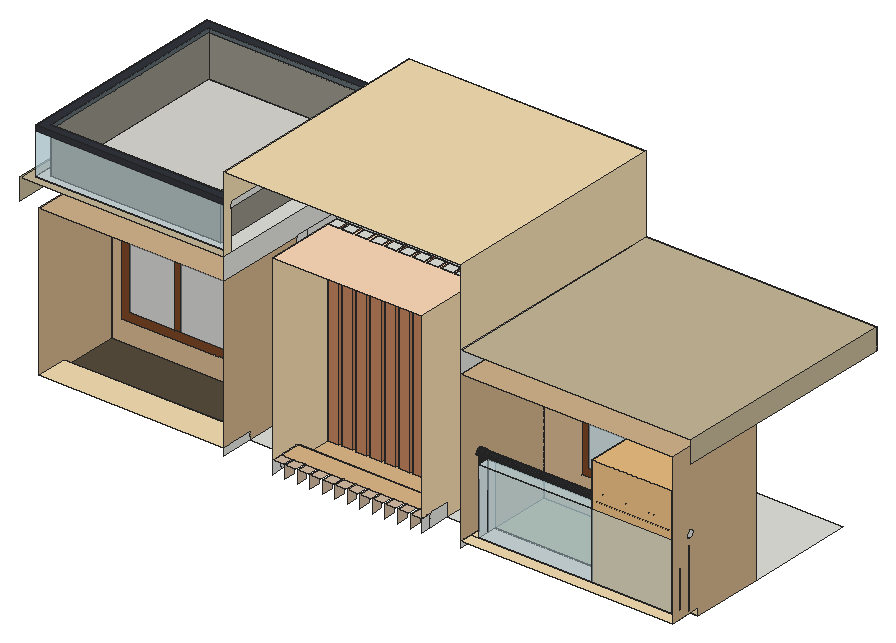
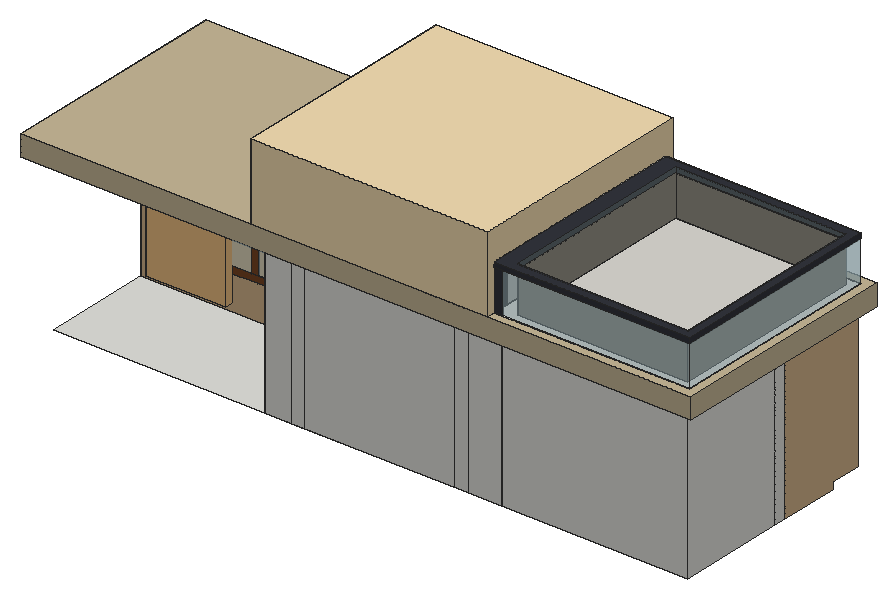
# SketchUp Ruby script. Lengths in inches.
U = 1.inch
M = Sketchup.active_model
def pt(a) = Geom::Point3d.new(a.map { |v| v * U })
def face(e, loops, mat)
  f = e.add_face(loops[0].map { |a| pt(a) })
  loops[1..].each { |l| e.add_face(l.map { |a| pt(a) }).erase! }
  f.material = f.back_material = mat if mat
  f
end
# faces: each face lists its corners as indices into pts; further lists are holes
def faces(e, pts, list, mat = nil) = list.each { |f| face(e, (f[0].is_a?(Array) ? f : [f]).map { |l| l.map { |i| pts[i] } }, mat) }
# xy, xz, yz: faces in a plane at the given z, y or x. An outline is a flat list of corners, or four numbers for a rectangle; further outlines are holes
def ring(l) = l.size == 4 ? [[l[0], l[1]], [l[2], l[1]], [l[2], l[3]], [l[0], l[3]]] : l.each_slice(2).to_a
def flat(e, list, mat, &to3) = list.each { |f| face(e, (f[0].is_a?(Array) ? f : [f]).map { |l| ring(l).map { |u, v| to3.(u, v) } }, mat) }
def xy(e, z, list, mat = nil) = flat(e, list, mat) { |x, y| [x, y, z] }
def xz(e, y, list, mat = nil) = flat(e, list, mat) { |x, z| [x, y, z] }
def yz(e, x, list, mat = nil) = flat(e, list, mat) { |y, z| [x, y, z] }
def lines(e, pts, list) = list.each { |a, b| e.add_line(pt(pts[a]), pt(pts[b])) }
# prism: a flat outline (further loops are holes) pulled along v
def prism(e, loops, v, mat = nil)
  f = face(e, loops, mat); d = Geom::Vector3d.new(v.map { |x| x * U })
  f.pushpull(f.normal.samedirection?(d) ? d.length : -d.length)
end
def box(e, o, s, mat = nil) = prism(e, [[o, [o[0] + s[0], o[1], o[2]], [o[0] + s[0], o[1] + s[1], o[2]], [o[0], o[1] + s[1], o[2]]]], [0, 0, s[2]], mat)
def at(x, y, z, deg = 0) = Geom::Transformation.translation(pt([x, y, z])) * Geom::Transformation.rotation(ORIGIN, Z_AXIS, deg.degrees)
def axes(o, x, y, z) = Geom::Transformation.new([*x, 0, *y, 0, *z, 0, *pt(o).to_a, 1])
def part(name) = M.definitions.add(name)
# library, detail: a bought-in or finely detailed component or shape, given as its bounding box
def library(name, o, s) = part(name).tap { |d| box(d.entities, o, s) }
def detail(e, o, s) = box(e.add_group.entities, o, s)
def put(e, d, t, mat = nil) = e.add_instance(d, t).tap { |i| i.material = mat if mat }
def group(e, t, mat = nil) = e.add_group.tap { |g| g.transformation = t; g.material = mat if mat }.entities
root = M.entities
M.materials.add("[0027_PeachPuff]").color = [255, 218, 185]
M.materials.add("[0034_Wheat]").color = [245, 222, 179]
M.materials.add("[0035_Tan]").color = [210, 180, 140]
M.materials.add("[0036_BurlyWood]1").color = [222, 184, 135]
M.materials.add("[Carpet Diamond Olive]").color = [87, 77, 61]
M.materials.add("[Formica Beige]").color = [247, 219, 174]
M.materials.add("[Formica Graystone]").color = [149, 146, 135]
M.materials.add("[Formica Laminate Dark]").color = [50, 53, 60]
M.materials.add("[Formica Laminate Light]").color = [213, 189, 164]
M.materials.add("[Formica Speckled Grey]").color = [94, 105, 111]
M.materials.add("[Quartz Light Brown]").color = [199, 184, 152]
M.materials.add("[Terrazzo Tile Light]").color = [219, 217, 210]
M.materials.add("[Tile Ceramic Natural]").color = [189, 180, 134]
M.materials.add("[Translucent Glass Gray]").color = [191, 191, 191]
M.materials["[Translucent Glass Gray]"].alpha = 0.5
M.materials.add("[Translucent Glass Safety]").color = [204, 235, 244]
M.materials["[Translucent Glass Safety]"].alpha = 0.5
M.materials.add("[Wood Veneer 01]").color = [120, 70, 37]
M.materials.add("[Wood Veneer 02]").color = [190, 128, 91]
c1 = library("chau cay",[-24.34,-109.24,0],[56.46,62.58,79.69])
xy(root,4500.3125,[[646.67,397.09,752.97,971.67],[752.97,397.09,800.41,971.67],[1272.8,397.09,1313.62,971.67],[1313.62,397.09,1398.32,971.67],[800.41,515.23,836.51,548.98],
  [842.91,515.23,879.01,548.98],[888.47,515.23,924.57,548.98],[934.66,515.23,970.76,548.98],[980.66,515.23,1016.76,548.98],[1024.6,515.23,1060.7,548.98],
  [1069.41,515.23,1105.51,548.98],[1113.97,515.23,1150.07,548.98],[1159.22,515.23,1195.32,548.98],[1202.41,515.23,1228.29,548.98],[1238.51,515.23,1272.8,548.98],
  [800.41,548.98,1272.8,971.67],[58.44,584.29,646.67,623.89],[58.44,623.89,646.67,971.67],[1398.32,623.89,2069.85,971.67]])
xy(root,4500.3125,[[800.41,397.09,1272.8,397.09,1272.8,515.23,1238.51,515.23,1238.51,548.98,1228.29,548.98,1228.29,515.23,1202.41,515.23,1202.41,548.98,1195.32,548.98,1195.32,515.23,1159.22,515.23,1159.22,548.98,1150.07,548.98,1150.07,515.23,1113.97,515.23,1113.97,548.98,1105.51,548.98,1105.51,515.23,1069.41,515.23,1069.41,548.98,1060.7,548.98,1060.7,515.23,1024.6,515.23,1024.6,548.98,1016.76,548.98,1016.76,515.23,980.66,515.23,980.66,548.98,970.76,548.98,970.76,515.23,934.66,515.23,934.66,548.98,924.57,548.98,924.57,515.23,888.47,515.23,888.47,548.98,879.01,548.98,879.01,515.23,842.91,515.23,842.91,548.98,836.51,548.98,836.51,515.23,800.41,515.23]],"[0036_BurlyWood]1")
xy(root,4500.3125,[[58.44,397.09,646.67,584.29]],"[Carpet Diamond Olive]")
xy(root,4500.3125,[[1398.32,397.09,2069.85,623.89]],"[Tile Ceramic Natural]")
xy(root,4522.25,[[1424.82,334.4,2037.625,397.09],[1412.33,356.37,1409.51,356.74,1406.89,357.82,1404.64,359.55,1402.91,361.8,1401.82,364.43,1401.45,367.24,1401.82,370.06,1402.91,372.68,1404.64,374.93,1406.89,376.66,1409.51,377.75,1412.33,378.12,1415.14,377.75,1417.76,376.66,1420.02,374.93,1421.74,372.68,1422.83,370.06,1423.2,367.24,1422.83,364.43,1421.74,361.8,1420.02,359.55,1417.76,357.82,1415.14,356.74],[2049.64,356.37,2046.82,356.74,2044.2,357.82,2041.95,359.55,2040.22,361.8,2039.13,364.43,2038.76,367.24,2039.13,370.06,2040.22,372.68,2041.95,374.93,2044.2,376.66,2046.82,377.75,2049.64,378.12,2052.45,377.75,2055.08,376.66,2057.33,374.93,2059.06,372.68,2060.14,370.06,2060.51,367.24,2060.14,364.43,2059.06,361.8,2057.33,359.55,2055.08,357.82,2052.45,356.74]])
xy(root,4522.25,[[58.44,295.82,646.67,397.09],[1398.32,295.82,2069.85,334.4],[[1398.32,334.4,1424.82,397.09],[1412.33,356.37,1409.51,356.74,1406.89,357.82,1404.64,359.55,1402.91,361.8,1401.82,364.43,1401.45,367.24,1401.82,370.06,1402.91,372.68,1404.64,374.93,1406.89,376.66,1409.51,377.75,1412.33,378.12,1415.14,377.75,1417.76,376.66,1420.02,374.93,1421.74,372.68,1422.83,370.06,1423.2,367.24,1422.83,364.43,1421.74,361.8,1420.02,359.55,1417.76,357.82,1415.14,356.74]],[[2037.625,334.4,2069.85,397.09],[2049.64,356.37,2046.82,356.74,2044.2,357.82,2041.95,359.55,2040.22,361.8,2039.13,364.43,2038.76,367.24,2039.13,370.06,2040.22,372.68,2041.95,374.93,2044.2,376.66,2046.82,377.75,2049.64,378.12,2052.45,377.75,2055.08,376.66,2057.33,374.93,2059.06,372.68,2060.14,370.06,2060.51,367.24,2060.14,364.43,2059.06,361.8,2057.33,359.55,2055.08,357.82,2052.45,356.74]]],"[0034_Wheat]")
xy(root,4541.3125,[[800.41,329.94,1272.8,397.09]],"[0036_BurlyWood]1")
xy(root,4541.3125,[[800.41,295.82,834.61,329.94],[840.03,295.82,874.24,329.94],[880.03,295.82,914.24,329.94],[919.91,295.82,954.11,329.94],[959.66,295.82,993.86,329.94],
  [998.72,295.82,1032.93,329.94],[1037.47,295.82,1071.68,329.94],[1076.91,295.82,1111.11,329.94],[1117.03,295.82,1151.24,329.94],[1157.28,295.82,1191.49,329.94],
  [1197.94,295.82,1232.15,329.94],[1238.6,295.82,1272.8,329.94]],"[Formica Laminate Light]")
xy(root,4730.6875,[[1424.82,334.4,2037.625,397.09]],"[Translucent Glass Safety]")
xy(root,4752.45,[[1412.33,356.37,1415.14,356.74,1417.76,357.82,1420.02,359.55,1421.74,361.8,1422.83,364.43,1423.2,367.24,1422.83,370.06,1421.74,372.68,1421.18,373.42,1403.47,373.42,1402.91,372.68,1401.82,370.06,1401.45,367.24,1401.82,364.43,1402.91,361.8,1404.64,359.55,1406.89,357.82,1409.51,356.74],[2049.64,356.37,2052.45,356.74,2055.08,357.82,2057.33,359.55,2059.06,361.8,2060.14,364.43,2060.51,367.24,2060.14,370.06,2059.06,372.68,2058.49,373.42,2040.79,373.42,2040.22,372.68,2039.13,370.06,2038.76,367.24,2039.13,364.43,2040.22,361.8,2041.95,359.55,2044.2,357.82,2046.82,356.74],[1403.47,373.42,1421.18,373.42,1420.02,374.93,1417.76,376.66,1415.14,377.75,1412.33,378.12,1409.51,377.75,1406.89,376.66,1404.64,374.93],[2040.79,373.42,2058.49,373.42,2057.33,374.93,2055.08,376.66,2052.45,377.75,2049.64,378.12,2046.82,377.75,2044.2,376.66,2041.95,374.93]])
xy(root,4996.25,[[58.44,584.29,646.67,623.89],[58.44,623.89,646.67,971.67]])
xy(root,4996.25,[[58.44,295.82,646.67,584.29],[1398.32,295.82,2069.85,623.89]],"[0035_Tan]")
xy(root,5063.875,[[[26.89,322.71,646.67,1003.22],[52.9375,348.75,593.74,977.17]],[646.67,971.67,752.97,1030.11],[752.97,971.67,800.41,1030.11],[800.41,971.67,1272.8,1030.11],[1272.8,971.67,1313.62,1030.11],
  [1313.62,971.67,1398.32,1030.11]])
xy(root,5063.875,[[0,295.82,646.67,295.82,646.67,322.71,26.89,322.71,26.89,1003.22,646.67,1003.22,646.67,1030.11,0,1030.11],[1398.32,295.82,2128.29,1030.11]],"[Quartz Light Brown]")
xy(root,5063.875,[[52.9375,348.75,593.74,977.17]],"[Terrazzo Tile Light]")
xy(root,5116.2,[[800.41,515.23,836.51,548.98],[842.91,515.23,879.01,548.98],[888.47,515.23,924.57,548.98],[934.66,515.23,970.76,548.98],[980.66,515.23,1016.76,548.98],
  [1024.6,515.23,1060.7,548.98],[1069.41,515.23,1105.51,548.98],[1113.97,515.23,1150.07,548.98],[1159.22,515.23,1195.32,548.98],[1202.41,515.23,1228.29,548.98],
  [1238.51,515.23,1272.8,548.98]])
xy(root,5116.2,[[800.41,295.82,800.41,515.23,836.51,515.23,836.51,548.98,842.91,548.98,842.91,515.23,879.01,515.23,879.01,548.98,888.47,548.98,888.47,515.23,924.57,515.23,924.57,548.98,934.66,548.98,934.66,515.23,970.76,515.23,970.76,548.98,980.66,548.98,980.66,515.23,1016.76,515.23,1016.76,548.98,1024.6,548.98,1024.6,515.23,1060.7,515.23,1060.7,548.98,1069.41,548.98,1069.41,515.23,1105.51,515.23,1105.51,548.98,1113.97,548.98,1113.97,515.23,1150.07,515.23,1150.07,548.98,1159.22,548.98,1159.22,515.23,1195.32,515.23,1195.32,548.98,1202.41,548.98,1202.41,515.23,1228.29,515.23,1228.29,548.98,1238.51,548.98,1238.51,515.23,1272.8,515.23,1272.8,295.82]],"[0027_PeachPuff]")
xy(root,5192.875,[[[26.89,322.71,646.67,1003.22],[52.9375,348.75,593.74,977.17]]])
xy(root,5209.125,[[[26.89,322.71,646.67,1003.22],[52.9375,348.75,593.74,977.17]]],"[Formica Laminate Dark]")
xy(root,5306.25,[[646.67,295.82,1398.32,1030.11]],"[0034_Wheat]")
xz(root,322.71,[[26.89,5192.875,646.67,5209.125]],"[Formica Laminate Dark]")
xz(root,322.71,[[26.89,5063.875,646.67,5192.875]],"[Translucent Glass Safety]")
xz(root,334.4,[[1424.82,4522.25,2037.625,4730.6875]],"[Translucent Glass Safety]")
xz(root,348.75,[[52.9375,5063.875,593.74,5192.875]],"[Formica Graystone]")
xz(root,348.75,[[52.9375,5192.875,593.74,5209.125]],"[Formica Speckled Grey]")
xz(root,397.09,[[58.44,4500.3125,646.67,4522.25],[1398.32,4500.3125,2069.85,4522.25]],"[0034_Wheat]")
xz(root,397.09,[[800.41,4500.3125,1272.8,4541.3125]],"[0036_BurlyWood]1")
xz(root,397.09,[[1424.82,4522.25,2037.625,4730.6875]],"[Translucent Glass Safety]")
xz(root,515.23,[[800.41,4500.3125,836.51,5116.2],[842.91,4500.3125,879.01,5116.2],[888.47,4500.3125,924.57,5116.2],[934.66,4500.3125,970.76,5116.2],[980.66,4500.3125,1016.76,5116.2],
  [1024.6,4500.3125,1060.7,5116.2],[1069.41,4500.3125,1105.51,5116.2],[1113.97,4500.3125,1150.07,5116.2],[1159.22,4500.3125,1195.32,5116.2],[1202.41,4500.3125,1228.29,5116.2],
  [1238.51,4500.3125,1272.8,5116.2]],"[Wood Veneer 02]")
xz(root,548.98,[[800.41,4500.3125,836.51,4996.25],[842.91,4500.3125,879.01,4996.25],[888.47,4500.3125,924.57,4996.25],[934.66,4500.3125,970.76,4996.25],[980.66,4500.3125,1016.76,4996.25],
  [1024.6,4500.3125,1060.7,4996.25],[1069.41,4500.3125,1105.51,4996.25],[1113.97,4500.3125,1150.07,4996.25],[1159.22,4500.3125,1195.32,4996.25],[1202.41,4500.3125,1228.29,4996.25],
  [1238.51,4500.3125,1272.8,4996.25],[800.41,4996.25,836.51,5116.2],[842.91,4996.25,879.01,5116.2],[888.47,4996.25,924.57,5116.2],[934.66,4996.25,970.76,5116.2],
  [980.66,4996.25,1016.76,5116.2],[1024.6,4996.25,1060.7,5116.2],[1069.41,4996.25,1105.51,5116.2],[1113.97,4996.25,1150.07,5116.2],[1159.22,4996.25,1195.32,5116.2],
  [1202.41,4996.25,1228.29,5116.2],[1238.51,4996.25,1272.8,5116.2]])
xz(root,548.98,[[836.51,4500.3125,842.91,5116.2],[879.01,4500.3125,888.47,5116.2],[924.57,4500.3125,934.66,5116.2],[970.76,4500.3125,980.66,5116.2],[1016.76,4500.3125,1024.6,5116.2],
  [1060.7,4500.3125,1069.41,5116.2],[1105.51,4500.3125,1113.97,5116.2],[1150.07,4500.3125,1159.22,5116.2],[1195.32,4500.3125,1202.41,5116.2],[1228.29,4500.3125,1238.51,5116.2]],"[Formica Laminate Dark]")
xz(root,584.29,[[[58.44,4500.3125,646.67,4996.25],[91.63,4567.02,618,4950.77]]],"[0035_Tan]")
xz(root,584.29,[[116.625,4592.01,260.25,4925.77],[279.73,4592.01,443.75,4925.77],[463.23,4592.01,593.01,4925.77]],"[Translucent Glass Gray]")
xz(root,584.29,[[[91.63,4567.02,618,4950.77],[116.625,4592.01,593.01,4925.77]],[260.25,4592.01,279.73,4925.77],[443.75,4592.01,463.23,4925.77]],"[Wood Veneer 01]")
xz(root,623.89,[[58.44,4500.3125,646.67,4996.25]])
xz(root,623.89,[[[1398.32,4500.3125,2069.85,4996.25],[1518.56,4608.64,1902.38,4947.7]]],"[0035_Tan]")
xz(root,623.89,[[1540.92,4631,1698.03,4925.34],[1719.28,4631,1880.02,4925.34]],"[Translucent Glass Safety]")
xz(root,623.89,[[[1518.56,4608.64,1902.38,4947.7],[1540.92,4631,1880.02,4925.34]],[1698.03,4631,1719.28,4925.34]],"[Wood Veneer 01]")
xz(root,971.67,[[58.44,4500.3125,646.67,4996.25],[646.67,4500.3125,752.97,4996.25],[752.97,4500.3125,800.41,4996.25],[800.41,4500.3125,1272.8,4996.25],[1272.8,4500.3125,1313.62,4996.25],
  [1313.62,4500.3125,1398.32,4996.25],[646.67,4996.25,752.97,5063.875],[752.97,4996.25,800.41,5063.875],[800.41,4996.25,1272.8,5063.875],[1272.8,4996.25,1313.62,5063.875],
  [1313.62,4996.25,1398.32,5063.875]])
xz(root,977.17,[[52.9375,5063.875,593.74,5192.875]],"[Formica Graystone]")
xz(root,977.17,[[52.9375,5192.875,593.74,5209.125]],"[Formica Speckled Grey]")
xz(root,1003.22,[[619.78,5063.875,646.67,5192.875],[26.89,5192.875,646.67,5209.125]],"[Formica Laminate Dark]")
xz(root,1003.22,[[26.89,5063.875,619.78,5192.875]],"[Translucent Glass Safety]")
xz(root,1030.11,[[646.67,5063.875,1398.32,5306.25]],"[0034_Wheat]")
xz(root,1030.11,[[0,4996.25,2128.29,5063.875]],"[Quartz Light Brown]")
yz(root,0,[[295.82,4996.25,1030.11,5063.875]],"[Quartz Light Brown]")
yz(root,26.89,[[322.71,5192.875,1003.22,5209.125]],"[Formica Laminate Dark]")
yz(root,26.89,[[322.71,5063.875,1003.22,5192.875]],"[Translucent Glass Safety]")
yz(root,52.9375,[[348.75,5063.875,977.17,5192.875]],"[Formica Graystone]")
yz(root,52.9375,[[348.75,5192.875,977.17,5209.125]],"[Formica Speckled Grey]")
yz(root,58.44,[[584.29,4500.3125,623.89,4996.25],[623.89,4500.3125,971.67,4996.25]])
yz(root,58.44,[[397.09,4500.3125,584.29,4500.3125,584.29,4996.25,295.82,4996.25,295.82,4522.25,397.09,4522.25]],"[0035_Tan]")
yz(root,593.74,[[348.75,5063.875,971.67,5192.875],[971.67,5063.875,977.17,5192.875],[971.67,5192.875,977.17,5209.125]],"[Formica Graystone]")
yz(root,593.74,[[348.75,5192.875,971.67,5209.125]],"[Formica Speckled Grey]")
yz(root,646.67,[[295.82,4500.3125,397.09,4522.25],[584.29,4500.3125,623.89,4996.25],[623.89,4500.3125,971.67,4996.25],[295.82,4996.25,971.67,5063.875],[322.71,5192.875,1003.22,5209.125]])
yz(root,646.67,[[295.82,5063.875,295.82,5306.25,1030.11,5306.25,1030.11,5063.875,1003.22,5063.875,1003.22,5209.125,322.71,5209.125,322.71,5063.875]],"[0034_Wheat]")
yz(root,646.67,[[397.09,4500.3125,397.09,4522.25,295.82,4522.25,295.82,4996.25,584.29,4996.25,584.29,4500.3125]],"[0035_Tan]")
yz(root,800.41,[[295.82,4500.3125,329.94,4541.3125],[329.94,4500.3125,397.09,4541.3125],[515.23,4500.3125,548.98,4996.25],[515.23,4996.25,548.98,5116.2]])
yz(root,800.41,[[397.09,4500.3125,515.23,4500.3125,515.23,5116.2,295.82,5116.2,295.82,4541.3125,397.09,4541.3125]],"[Formica Beige]")
yz(root,836.51,[[515.23,4500.3125,548.98,4996.25],[515.23,4996.25,548.98,5116.2]],"[Wood Veneer 02]")
yz(root,840.03,[[295.82,4500.3125,329.94,4541.3125]],"[Formica Laminate Light]")
yz(root,842.91,[[515.23,4500.3125,548.98,4996.25],[515.23,4996.25,548.98,5116.2]])
yz(root,879.01,[[515.23,4500.3125,548.98,4996.25],[515.23,4996.25,548.98,5116.2]],"[Wood Veneer 02]")
yz(root,880.03,[[295.82,4500.3125,329.94,4541.3125]],"[Formica Laminate Light]")
yz(root,888.47,[[515.23,4500.3125,548.98,4996.25],[515.23,4996.25,548.98,5116.2]],"[Wood Veneer 02]")
yz(root,919.91,[[295.82,4500.3125,329.94,4541.3125]],"[Formica Laminate Light]")
yz(root,924.57,[[515.23,4500.3125,548.98,4996.25],[515.23,4996.25,548.98,5116.2]],"[Wood Veneer 02]")
yz(root,934.66,[[515.23,4500.3125,548.98,4996.25],[515.23,4996.25,548.98,5116.2]],"[Wood Veneer 02]")
yz(root,959.66,[[295.82,4500.3125,329.94,4541.3125]],"[Formica Laminate Light]")
yz(root,970.76,[[515.23,4500.3125,548.98,4996.25],[515.23,4996.25,548.98,5116.2]],"[Wood Veneer 02]")
yz(root,980.66,[[515.23,4500.3125,548.98,4996.25],[515.23,4996.25,548.98,5116.2]],"[Wood Veneer 02]")
yz(root,998.72,[[295.82,4500.3125,329.94,4541.3125]],"[Formica Laminate Light]")
yz(root,1016.76,[[515.23,4500.3125,548.98,4996.25],[515.23,4996.25,548.98,5116.2]],"[Wood Veneer 02]")
yz(root,1024.6,[[515.23,4500.3125,548.98,4996.25],[515.23,4996.25,548.98,5116.2]],"[Wood Veneer 02]")
yz(root,1037.47,[[295.82,4500.3125,329.94,4541.3125]],"[Formica Laminate Light]")
yz(root,1060.7,[[515.23,4500.3125,548.98,4996.25],[515.23,4996.25,548.98,5116.2]],"[Wood Veneer 02]")
yz(root,1069.41,[[515.23,4500.3125,548.98,4996.25],[515.23,4996.25,548.98,5116.2]],"[Wood Veneer 02]")
yz(root,1076.91,[[295.82,4500.3125,329.94,4541.3125]],"[Formica Laminate Light]")
yz(root,1105.51,[[515.23,4500.3125,548.98,4996.25],[515.23,4996.25,548.98,5116.2]],"[Wood Veneer 02]")
yz(root,1113.97,[[515.23,4500.3125,548.98,4996.25],[515.23,4996.25,548.98,5116.2]],"[Wood Veneer 02]")
yz(root,1117.03,[[295.82,4500.3125,329.94,4541.3125]],"[Formica Laminate Light]")
yz(root,1150.07,[[515.23,4500.3125,548.98,4996.25],[515.23,4996.25,548.98,5116.2]],"[Wood Veneer 02]")
yz(root,1157.28,[[295.82,4500.3125,329.94,4541.3125]],"[Formica Laminate Light]")
yz(root,1159.22,[[515.23,4500.3125,548.98,4996.25],[515.23,4996.25,548.98,5116.2]],"[Wood Veneer 02]")
yz(root,1195.32,[[515.23,4500.3125,548.98,4996.25],[515.23,4996.25,548.98,5116.2]],"[Wood Veneer 02]")
yz(root,1197.94,[[295.82,4500.3125,329.94,4541.3125]],"[Formica Laminate Light]")
yz(root,1202.41,[[515.23,4500.3125,548.98,4996.25],[515.23,4996.25,548.98,5116.2]],"[Wood Veneer 02]")
yz(root,1228.29,[[515.23,4500.3125,548.98,4996.25],[515.23,4996.25,548.98,5116.2]],"[Wood Veneer 02]")
yz(root,1238.51,[[515.23,4500.3125,548.98,4996.25],[515.23,4996.25,548.98,5116.2]],"[Wood Veneer 02]")
yz(root,1238.6,[[295.82,4500.3125,329.94,4541.3125]],"[Formica Laminate Light]")
yz(root,1272.8,[[295.82,4500.3125,329.94,4541.3125],[329.94,4500.3125,397.09,4541.3125],[515.23,4500.3125,548.98,4996.25],[515.23,4996.25,548.98,5116.2]])
yz(root,1272.8,[[397.09,4500.3125,397.09,4541.3125,295.82,4541.3125,295.82,5116.2,515.23,5116.2,515.23,4500.3125]],"[Formica Beige]")
yz(root,1398.32,[[295.82,4500.3125,397.09,4522.25],[623.89,4500.3125,971.67,4996.25],[295.82,4996.25,971.67,5063.875]])
yz(root,1398.32,[[295.82,5063.875,1030.11,5306.25]],"[0034_Wheat]")
yz(root,1398.32,[[[397.09,4500.3125,623.89,4500.3125,623.89,4996.25,295.82,4996.25,295.82,4522.25,397.09,4522.25],[364,4736.14,361.19,4736.51,358.5625,4737.6,356.31,4739.33,354.58,4741.58,353.5,4744.2,353.125,4747.02,353.5,4749.83,354.58,4752.45,356.31,4754.71,358.5625,4756.43,361.19,4757.52,364,4757.89,366.81,4757.52,369.4375,4756.43,371.69,4754.71,373.42,4752.45,374.5,4749.83,374.875,4747.02,374.5,4744.2,373.42,4741.58,371.69,4739.33,369.4375,4737.6,366.81,4736.51]]],"[0035_Tan]")
yz(root,1424.82,[[334.4,4522.25,397.09,4730.6875]])
yz(root,2037.625,[[334.4,4522.25,397.09,4730.6875]])
yz(root,2069.85,[[364,4736.14,366.81,4736.51,369.4375,4737.6,371.69,4739.33,373.42,4741.58,374.5,4744.2,374.875,4747.02,374.5,4749.83,373.42,4752.45,371.69,4754.71,369.4375,4756.43,366.81,4757.52,364,4757.89,361.19,4757.52,358.5625,4756.43,356.31,4754.71,354.58,4752.45,353.5,4749.83,353.125,4747.02,353.5,4744.2,354.58,4741.58,356.31,4739.33,358.5625,4737.6,361.19,4736.51]])
yz(root,2069.85,[[[397.09,4500.3125,397.09,4522.25,295.82,4522.25,295.82,4996.25,623.89,4996.25,623.89,4500.3125],[364,4736.14,366.81,4736.51,369.4375,4737.6,371.69,4739.33,373.42,4741.58,374.5,4744.2,374.875,4747.02,374.5,4749.83,373.42,4752.45,371.69,4754.71,369.4375,4756.43,366.81,4757.52,364,4757.89,361.19,4757.52,358.5625,4756.43,356.31,4754.71,354.58,4752.45,353.5,4749.83,353.125,4747.02,353.5,4744.2,354.58,4741.58,356.31,4739.33,358.5625,4737.6,361.19,4736.51]]],"[0035_Tan]")
yz(root,2128.29,[[295.82,4996.25,1030.11,5063.875]],"[Quartz Light Brown]")
p = [[1409.51,356.74,4522.25],[1412.33,356.37,4522.25],[1412.33,356.37,4752.45],[1409.51,356.74,4752.45],[1415.14,356.74,4522.25],[1415.14,356.74,4752.45],
  [2046.82,356.74,4522.25],[2049.64,356.37,4522.25],[2049.64,356.37,4752.45],[2046.82,356.74,4752.45],[2052.45,356.74,4522.25],[2052.45,356.74,4752.45],
  [1406.89,357.82,4522.25],[1406.89,357.82,4752.45],[1417.76,357.82,4522.25],[1417.76,357.82,4752.45],[2044.2,357.82,4522.25],[2044.2,357.82,4752.45],
  [2055.08,357.82,4522.25],[2055.08,357.82,4752.45],[1404.64,359.55,4522.25],[1404.64,359.55,4752.45],[1420.02,359.55,4522.25],[1420.02,359.55,4752.45],
  [2041.95,359.55,4522.25],[2041.95,359.55,4752.45],[2057.33,359.55,4522.25],[2057.33,359.55,4752.45],[1402.91,361.8,4522.25],[1402.91,361.8,4752.45],
  [1421.74,361.8,4522.25],[1421.74,361.8,4752.45],[2040.22,361.8,4522.25],[2040.22,361.8,4752.45],[2059.06,361.8,4522.25],[2059.06,361.8,4752.45],
  [1401.82,364.43,4522.25],[1401.82,364.43,4752.45],[1422.83,364.43,4522.25],[1422.83,364.43,4752.45],[2039.13,364.43,4522.25],[2039.13,364.43,4752.45],
  [2060.14,364.43,4522.25],[2060.14,364.43,4752.45],[1401.45,367.24,4522.25],[1401.45,367.24,4752.45],[1423.2,367.24,4522.25],[1423.2,367.24,4752.45],
  [2038.76,367.24,4522.25],[2038.76,367.24,4752.45],[2060.51,367.24,4522.25],[2060.51,367.24,4752.45],[1401.82,370.06,4522.25],[1401.82,370.06,4752.45],
  [1422.83,370.06,4522.25],[1422.83,370.06,4752.45],[2039.13,370.06,4522.25],[2039.13,370.06,4752.45],[2060.14,370.06,4522.25],[2060.14,370.06,4752.45],
  [1402.91,372.68,4522.25],[1402.91,372.68,4752.45],[1421.74,372.68,4522.25],[1421.74,372.68,4752.45],[2040.22,372.68,4522.25],[2040.22,372.68,4752.45],
  [2059.06,372.68,4522.25],[2059.06,372.68,4752.45],[1404.64,374.93,4522.25],[1403.47,373.42,4752.45],[1404.64,374.93,4752.45],[1420.02,374.93,4522.25],
  [1420.02,374.93,4752.45],[1421.18,373.42,4752.45],[2041.95,374.93,4522.25],[2040.79,373.42,4752.45],[2041.95,374.93,4752.45],[2057.33,374.93,4522.25],
  [2057.33,374.93,4752.45],[2058.49,373.42,4752.45],[1406.89,376.66,4522.25],[1406.89,376.66,4752.45],[1417.76,376.66,4522.25],[1417.76,376.66,4752.45],
  [2044.2,376.66,4522.25],[2044.2,376.66,4752.45],[2055.08,376.66,4522.25],[2055.08,376.66,4752.45],[1409.51,377.75,4522.25],[1409.51,377.75,4752.45],
  [1415.14,377.75,4522.25],[1415.14,377.75,4752.45],[2046.82,377.75,4522.25],[2046.82,377.75,4752.45],[2052.45,377.75,4522.25],[2052.45,377.75,4752.45],
  [1412.33,378.12,4522.25],[1412.33,378.12,4752.45],[2049.64,378.12,4522.25],[2049.64,378.12,4752.45],[2069.85,364,4736.14],[2069.85,361.19,4736.51],
  [1398.32,361.19,4736.51],[1398.32,364,4736.14],[2069.85,366.81,4736.51],[1398.32,366.81,4736.51],[2069.85,358.5625,4737.6],[1398.32,358.5625,4737.6],
  [2069.85,369.4375,4737.6],[1398.32,369.4375,4737.6],[2069.85,356.31,4739.33],[1398.32,356.31,4739.33],[2069.85,371.69,4739.33],[1398.32,371.69,4739.33],
  [2069.85,354.58,4741.58],[1398.32,354.58,4741.58],[2069.85,373.42,4741.58],[1398.32,373.42,4741.58],[2069.85,353.5,4744.2],[1398.32,353.5,4744.2],
  [2069.85,374.5,4744.2],[1398.32,374.5,4744.2],[2069.85,353.125,4747.02],[1398.32,353.125,4747.02],[2069.85,374.875,4747.02],[1398.32,374.875,4747.02],
  [2069.85,353.5,4749.83],[1398.32,353.5,4749.83],[2069.85,374.5,4749.83],[1398.32,374.5,4749.83],[2069.85,354.58,4752.45],[1398.32,354.58,4752.45],
  [2069.85,373.42,4752.45],[1398.32,373.42,4752.45],[2069.85,356.31,4754.71],[1398.32,356.31,4754.71],[2069.85,371.69,4754.71],[1398.32,371.69,4754.71],
  [2069.85,358.5625,4756.43],[1398.32,358.5625,4756.43],[2069.85,369.4375,4756.43],[1398.32,369.4375,4756.43],[2069.85,361.19,4757.52],[1398.32,361.19,4757.52],
  [2069.85,366.81,4757.52],[1398.32,366.81,4757.52],[2069.85,364,4757.89],[1398.32,364,4757.89],[800.41,548.98,5159.08],[800.41,971.67,5159.08],
  [1272.8,548.98,5159.08],[1272.8,971.67,5159.08],[800.41,548.98,5116.2],[1272.8,548.98,5116.2]]
faces(root,p,[[0,1,2,3],[1,4,5,2],[6,7,8,9],[7,10,11,8],[12,0,3,13],[4,14,15,5],[16,6,9,17],[10,18,19,11],
  [20,12,13,21],[14,22,23,15],[24,16,17,25],[18,26,27,19],[28,20,21,29],[22,30,31,23],[32,24,25,33],[26,34,35,27],
  [36,28,29,37],[30,38,39,31],[40,32,33,41],[34,42,43,35],[44,36,37,45],[38,46,47,39],[48,40,41,49],[42,50,51,43],
  [52,44,45,53],[46,54,55,47],[56,48,49,57],[50,58,59,51],[60,52,53,61],[54,62,63,55],[64,56,57,65],[58,66,67,59],
  [68,60,61,69,70],[62,71,72,73,63],[74,64,65,75,76],[66,77,78,79,67],[80,68,70,81],[71,82,83,72],[84,74,76,85],[77,86,87,78],
  [88,80,81,89],[82,90,91,83],[92,84,85,93],[86,94,95,87],[96,88,89,97],[90,96,97,91],[98,92,93,99],[94,98,99,95],
  [100,101,102,103],[104,100,103,105],[101,106,107,102],[108,104,105,109],[106,110,111,107],[112,108,109,113],[110,114,115,111],[116,112,113,117],
  [114,118,119,115],[120,116,117,121],[118,122,123,119],[124,120,121,125],[122,126,127,123],[128,124,125,129],[126,130,131,127],[132,128,129,133,69,73,75,79],
  [130,134,135,131],[136,132,79,75,73,69,133,137],[134,138,139,135],[140,136,137,141],[138,142,143,139],[144,140,141,145],[142,146,147,143],[146,144,145,147]],"[Formica Laminate Dark]")
lines(root,p,[[148,149],[150,151],[148,152],[150,153]])
put(root,c1,axes([1893.09,102.75,4522.25],[4.5,0,0],[0,-4.9651,0],[0,0,4.37432]))
